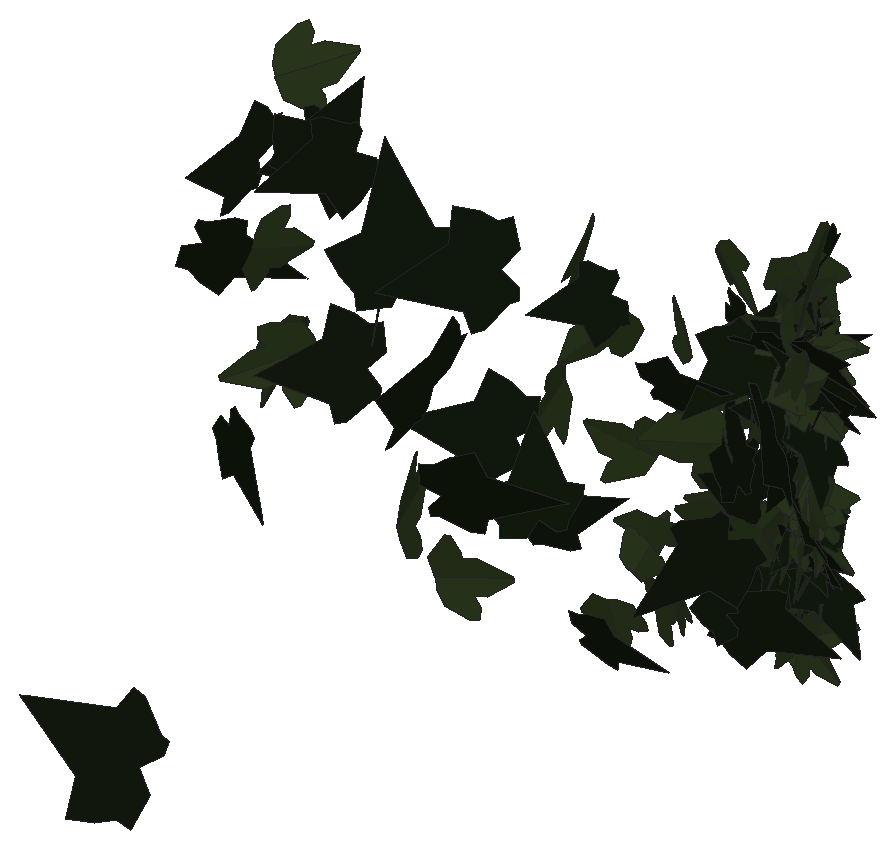
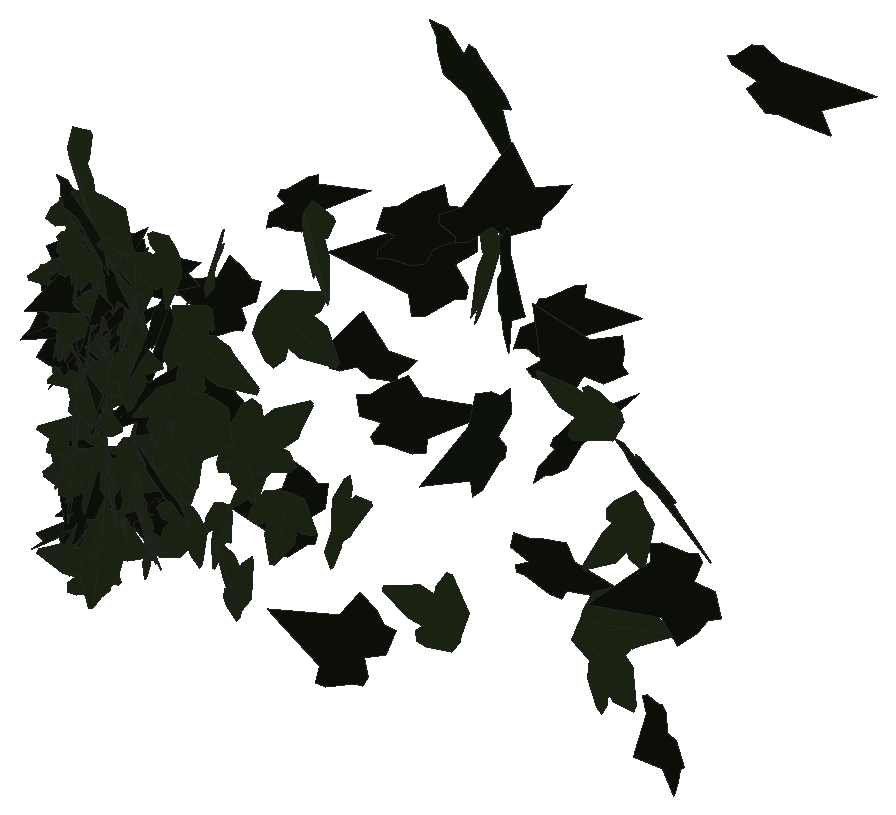
# SketchUp Ruby script. Lengths in inches.
U = 1.inch
M = Sketchup.active_model
def pt(a) = Geom::Point3d.new(a.map { |v| v * U })
def face(e, loops, mat)
  f = e.add_face(loops[0].map { |a| pt(a) })
  loops[1..].each { |l| e.add_face(l.map { |a| pt(a) }).erase! }
  f.material = f.back_material = mat if mat
  f
end
# faces: each face lists its corners as indices into pts; further lists are holes
def faces(e, pts, list, mat = nil) = list.each { |f| face(e, (f[0].is_a?(Array) ? f : [f]).map { |l| l.map { |i| pts[i] } }, mat) }
# xy, xz, yz: faces in a plane at the given z, y or x. An outline is a flat list of corners, or four numbers for a rectangle; further outlines are holes
def ring(l) = l.size == 4 ? [[l[0], l[1]], [l[2], l[1]], [l[2], l[3]], [l[0], l[3]]] : l.each_slice(2).to_a
def flat(e, list, mat, &to3) = list.each { |f| face(e, (f[0].is_a?(Array) ? f : [f]).map { |l| ring(l).map { |u, v| to3.(u, v) } }, mat) }
def xy(e, z, list, mat = nil) = flat(e, list, mat) { |x, y| [x, y, z] }
def xz(e, y, list, mat = nil) = flat(e, list, mat) { |x, z| [x, y, z] }
def yz(e, x, list, mat = nil) = flat(e, list, mat) { |y, z| [x, y, z] }
def lines(e, pts, list) = list.each { |a, b| e.add_line(pt(pts[a]), pt(pts[b])) }
# prism: a flat outline (further loops are holes) pulled along v
def prism(e, loops, v, mat = nil)
  f = face(e, loops, mat); d = Geom::Vector3d.new(v.map { |x| x * U })
  f.pushpull(f.normal.samedirection?(d) ? d.length : -d.length)
end
def box(e, o, s, mat = nil) = prism(e, [[o, [o[0] + s[0], o[1], o[2]], [o[0] + s[0], o[1] + s[1], o[2]], [o[0], o[1] + s[1], o[2]]]], [0, 0, s[2]], mat)
def at(x, y, z, deg = 0) = Geom::Transformation.translation(pt([x, y, z])) * Geom::Transformation.rotation(ORIGIN, Z_AXIS, deg.degrees)
def axes(o, x, y, z) = Geom::Transformation.new([*x, 0, *y, 0, *z, 0, *pt(o).to_a, 1])
def part(name) = M.definitions.add(name)
# library, detail: a bought-in or finely detailed component or shape, given as its bounding box
def library(name, o, s) = part(name).tap { |d| box(d.entities, o, s) }
def detail(e, o, s) = box(e.add_group.entities, o, s)
def put(e, d, t, mat = nil) = e.add_instance(d, t).tap { |i| i.material = mat if mat }
def group(e, t, mat = nil) = e.add_group.tap { |g| g.transformation = t; g.material = mat if mat }.entities
root = M.entities
M.materials.add("efeu1").color = [18, 25, 13]
M.materials.add("efeu2").color = [43, 57, 29]
c1 = part("ivyleaf_9")
p = [[1.54,2.16,1.25],[1.36,2.04,1.19],[-0.21,0.99,0.68],[-0.71,1.11,0.82],[-0.85,0.86,0.67],[-0.8,0.17,0.21],
  [-0.9,-0.01,0.1],[-0.67,-0.16,-0.02],[-0.08,-0.08,-0.05],[-0.03,-0.6,-0.4],[0.65,-0.88,-0.66],[0.83,-0.6,-0.49],
  [1.29,-0.42,-0.43],[1.8125,-0.07,-0.26],[1.21,0.44,0.15]]
faces(c1.entities,p,[[0,1,2,3,4,5,6,7,8,9,10,11,12,13,14]],"efeu1")
c2 = part("ivyleaf_10")
p = [[0,0.5,-0.03],[-0.0625,2.02,-0.43],[-0.19,2.01,-0.46],[-0.54,1.05,-0.29],[-0.52,0.625,-0.18],[-0.83,0.76,-0.28],
  [-1.16,0.64,-0.33],[-1.15,0.33,-0.24],[-0.77,-0.39,0.02],[-0.3,-0.51,0.16],[0.04,-0.48,0.23],[-0.02,2.01,-0.4375],
  [-0.06,2.01,-0.43],[0.04,-0.49,0.23],[0.67,-0.49,0.14],[1.38,0.36,-0.2],[1.375,0.51,-0.24],[0.81,0.65,-0.19],
  [0.62,0.59,-0.15],[0.6,1.09,-0.28],[0.5,1.23,-0.31]]
faces(c2.entities,p,[[0,1,2,3,4,5,6,7,8,9,10],[11,12,0,13,14,15,16,17,18,19,20]],"efeu2")
put(root,c1,axes([582.17,102.53,177.91],[-0.93537,-0.48465,-0.89648],[-0.80042,-0.4038,1.05345],[-0.63079,1.23107,-0.00739]))
put(root,c1,axes([582.29,115.48,184.26],[-0.73247,1.14725,0.43552],[-0.25175,0.35593,-1.361],[-1.20104,-0.77428,0.01967]))
put(root,c2,axes([580.5,116.68,178.94],[-0.03504,0.01507,1.25714],[-0.80764,0.96354,-0.03406],[-0.96351,-0.80822,-0.01717]))
put(root,c1,axes([580.96,117.87,179.3],[0.6414,0.06722,0.97347],[0.97264,0.04951,-0.64427],[-0.07836,1.16473,-0.02879]))
put(root,c1,axes([576.85,121.08,183.4375],[-0.9038,-0.73638,0.60147],[0.47307,0.37156,1.16577],[-0.82475,1.02008,0.00956]))
put(root,c1,axes([581.51,121.23,177.39],[-0.91994,-0.16178,0.29692],[0.29433,0.04052,0.934],[-0.16644,0.96582,0.01055]))
put(root,c1,axes([578.58,123.02,183.34],[-0.59552,-0.39328,0.97343],[-0.81155,-0.53754,-0.71367],[0.66605,-1.00661,0.00079]))
put(root,c1,axes([574.84,123.16,183.46],[-0.4066,0.16227,-1.11029],[1.00642,-0.46946,-0.43717],[-0.49618,-1.0852,0.0231]))
put(root,c1,axes([582.08,122.8,173.05],[0.59099,-0.20629,0.62747],[0.59502,-0.19926,-0.62594],[0.28676,0.83862,0.00563]))
put(root,c1,axes([581.98,123.71,183.42],[-0.03674,-0.4484,-0.69223],[-0.05769,-0.68983,0.4499],[-0.82275,0.06839,-0.00063]))
put(root,c1,axes([578.5,123.73,177.73],[-0.46486,-0.0952,0.97458],[-0.95808,-0.17874,-0.47445],[0.20237,-1.06487,-0.00749]))
put(root,c1,axes([585.64,124.3,176.6],[-0.0035,0.04747,-1.11243],[-0.00157,-1.11244,-0.04746],[-1.11344,0.00142,0.00356]))
put(root,c2,axes([582.25,123.57,173.63],[-0.82414,-0.10409,-0.03694],[0.03705,0.00142,-0.83069],[0.10405,-0.82497,0.00323]))
put(root,c2,axes([576.16,123.99,172.28],[-0.30247,-0.08255,0.97235],[0.90328,0.36153,0.31168],[-0.36927,0.95197,-0.03405]))
put(root,c1,axes([571.91,124.95,183.84],[-0.02923,-0.38443,-0.92473],[-0.056,-0.92304,0.3855],[-0.99988,0.06294,0.00544]))
put(root,c2,axes([582.64,124.8,175.91],[-0.65772,-0.30074,0.20225],[-0.18186,-0.08863,-0.7232],[0.3135,-0.68238,0.0048]))
put(root,c2,axes([580.02,125.125,183.85],[0.45167,-0.99129,0.04723],[0.02824,-0.03903,-1.0893],[0.99201,0.45246,0.00951]))
put(root,c2,axes([582.47,124.46,174.89],[0.20307,0.44166,-0.59525],[0.20821,0.55835,0.4853],[0.71136,-0.2895,0.02788]))
put(root,c1,axes([582.85,124.88,180.375],[0.3547,-0.07925,0.67611],[0.66329,-0.13123,-0.36336],[0.1531,0.75213,0.00784]))
put(root,c1,axes([585.99,126.1,179.18],[0.06523,-0.507,1.17159],[0.16337,-1.16015,-0.51115],[1.26609,0.17582,0.0056]))
put(root,c2,axes([584.38,125.29,178.92],[-0.32504,0.07068,1.22055],[-1.18819,-0.31576,-0.29813],[0.28799,-1.22298,0.14751]))
put(root,c1,axes([585.21,125.39,173.81],[-0.343,-0.79962,0.40835],[0.17244,0.37033,0.87001],[-0.88114,0.38374,0.01131]))
put(root,c2,axes([580.57,125.81,181.18],[-0.41497,-0.51387,0.77483],[-0.48662,-0.60297,-0.66051],[0.79224,-0.63953,0.00015]))
put(root,c2,axes([583.1,125.24,173.72],[-0.6164,0.35233,0.11163],[-0.09557,0.05773,-0.70999],[-0.35702,-0.62376,-0.00266]))
put(root,c1,axes([571.65,125.78,176.58],[-0.85339,0.08103,0.70567],[-0.70238,0.06808,-0.85723],[-0.10583,-1.10527,-0.00107]))
put(root,c1,axes([570.375,125.24,182.8],[-0.58712,-0.05013,0.79979],[0.79707,0.06588,0.58926],[-0.08277,0.98997,0.00129]))
put(root,c2,axes([583.26,125.53,181.48],[-0.39235,0.6292,-0.08563],[-0.05289,0.06793,0.74145],[0.63279,0.3958,0.00888]))
put(root,c1,axes([585.23,125.36,178.03],[-0.1394,-0.60796,0.74109],[0.15988,0.72365,0.62372],[-0.94512,0.21208,-0.0038]))
put(root,c1,axes([585.57,125.2,173.91],[0.10177,0.10772,-0.99977],[0.48767,0.87351,0.14376],[0.87939,-0.49687,0.03598]))
put(root,c1,axes([566.9,125.91,172.87],[-0.18101,-0.05084,-0.95511],[0.94753,0.12305,-0.18612],[0.13046,-0.96429,0.02661]))
put(root,c2,axes([581.23,126.19,177.14],[-0.43596,-0.29641,-0.80312],[-0.66848,-0.44515,0.52716],[-0.53479,0.79806,-0.00425]))
put(root,c2,axes([568.93,126.3,175.9],[0.28392,0.20306,-1.03576],[-0.84049,-0.60529,-0.34906],[-0.63844,0.88715,-0.00108]))
put(root,c2,axes([584.6,125.74,176.125],[-1.12151,-0.23936,0.38892],[-0.38144,-0.07608,-1.14676],[0.25111,-1.18459,-0.00493]))
put(root,c1,axes([584.91,126.36,181.38],[-0.70613,-0.48878,0.24061],[-0.19812,-0.13654,-0.85879],[0.50749,-0.7334,-0.00047]))
put(root,c1,axes([584.99,126.55,176.8],[0.03301,0.04778,0.85129],[-0.62056,-0.58288,0.05678],[0.58471,-0.62132,0.0122]))
put(root,c2,axes([581.64,126.35,172.23],[-0.47915,0.12037,0.77564],[0.75107,-0.19371,0.49403],[0.22805,0.89089,0.00262]))
put(root,c2,axes([583.87,126.32,176.32],[-0.49622,-0.36773,0.31232],[-0.25775,-0.17668,-0.61753],[0.40784,-0.55907,-0.01027]))
put(root,c2,axes([584.49,126.83,173],[-0.12467,0.23622,-0.59228],[0.0462,-0.59856,-0.24845],[-0.63597,-0.08979,0.09805]))
put(root,c2,axes([568.09,125.8125,179.2],[-0.13983,-0.38674,-0.93422],[0.31512,0.87947,-0.41125],[0.96075,-0.34475,-0.00108]))
put(root,c2,axes([584.65,126.98,179.65],[-0.08804,0.30993,-0.6085],[0.1578,-0.5877,-0.32217],[-0.6644,-0.18065,0.00412]))
put(root,c1,axes([567.35,126.4,181.41],[-0.82327,0.75225,0.36065],[-0.29416,0.21237,-1.11449],[-0.78065,-0.87335,0.03962]))
put(root,c1,axes([572.34,126.67,180.68],[0.98632,-0.53087,0.11326],[0.09969,-0.05374,-1.12011],[0.53359,0.99135,-0.00007]))
put(root,c1,axes([569.29,127.62,181.86],[0.2206,-0.71775,-0.75354],[0.2562,-0.70912,0.75044],[-1.00864,-0.3371,0.02581]))
put(root,c1,axes([565.74,126.29,178.21],[0.16963,0.21121,-0.96973],[0.50806,0.82663,0.26891],[0.85256,-0.53463,0.03269]))
put(root,c2,axes([585.58,127.33,172.43],[-0.20273,0.3687,0.76453],[0.34712,-0.68129,0.4206],[0.77457,0.40181,0.01162]))
put(root,c1,axes([584.92,126.46,181.77],[0.67205,0.44331,-0.09212],[-0.08109,-0.04436,-0.80505],[-0.44546,0.67688,0.00757]))
put(root,c2,axes([584.93,127.31,175.88],[-0.07555,-0.4841,0.51265],[-0.08314,-0.50587,-0.48995],[0.70017,-0.1123,-0.00286]))
put(root,c1,axes([585.2,127.7,178.13],[0.34566,-0.34734,-1.02118],[0.843,-0.58198,0.4833],[-0.67291,-0.90751,0.08091]))
put(root,c2,axes([584.92,127.38,173.9],[-0.11298,-0.21399,-0.59135],[0.18528,-0.58548,0.17647],[-0.60097,-0.14027,0.16557]))
put(root,c2,axes([567.78,127.5,175.56],[0.14329,-0.90028,0.5439],[0.13463,-0.52871,-0.91061],[1.04317,0.1919,0.04281]))
put(root,c1,axes([585.65,127.68,179.2],[-0.21749,-0.09841,0.81849],[-0.56861,-0.59501,-0.22263],[0.59691,-0.60266,0.08615]))
put(root,c1,axes([585.92,127.54,176.01],[0.51861,-0.26683,-0.50331],[0.45478,-0.21599,0.58311],[-0.34308,-0.68966,0.01212]))
put(root,c2,axes([576.98,127.84,176.83],[0.00492,0.27558,-1.00343],[-0.01675,-1.00329,-0.27563],[-1.04045,0.01745,-0.00031]))
put(root,c2,axes([584.75,127.12,181.93],[-0.65202,-0.36991,0.09537],[-0.08279,-0.04733,-0.74964],[0.37293,-0.65725,0.00031]))
put(root,c2,axes([584.76,127.26,180.35],[-0.31984,0.04707,-0.60666],[0.55158,-0.26698,-0.31151],[-0.25695,-0.63171,0.08645]))
put(root,c2,axes([585.33,127.53,179.35],[0.18007,-0.1421,0.66759],[0.51689,-0.42252,-0.22935],[0.44576,0.54734,-0.00373]))
put(root,c2,axes([586.35,127.55,184.8],[0.71848,-0.97219,0.35474],[0.20971,-0.28612,-1.20887],[1.01342,0.74846,-0.00135]))
put(root,c2,axes([585.73,127.67,174.77],[0.23607,-0.28493,0.63083],[0.41476,-0.47539,-0.36993],[0.55418,0.47716,0.00814]))
put(root,c2,axes([586.13,127.22,181.3125],[0.01819,-0.89941,-0.16555],[0.08683,0.16653,-0.89521],[0.91038,0.00208,0.08869]))
put(root,c2,axes([584.9,127.24,174.82],[-0.60543,0.32042,-0.18819],[-0.16626,0.08815,0.68499],[0.33232,0.62784,-0.00014]))
put(root,c2,axes([586.0625,127.58,176.98],[0.3499,-0.27622,-0.70319],[0.53936,-0.4513,0.44566],[-0.52902,-0.64283,-0.01072]))
put(root,c2,axes([585.3,126.8,181.07],[0.35422,-0.11,-1.10319],[1.01416,0.50003,0.27578],[0.44789,-1.04521,0.24803]))
put(root,c1,axes([586.17,127.74,178.76],[0.07757,-0.79632,0.18314],[0.08695,-0.17488,-0.79721],[0.81247,0.09474,0.06784]))
put(root,c1,axes([585.55,127.76,174.05],[-0.6011,-0.61068,-0.00073],[0.00064,0.00039,-0.85688],[0.61068,-0.6011,0.00019]))
put(root,c2,axes([585.8,127.43,172.24],[0.23437,-0.07647,0.87599],[0.87838,-0.02155,-0.23689],[0.04065,0.90654,0.06827]))
put(root,c1,axes([586.11,127.72,181.13],[0.04619,0.09351,0.82911],[-0.75499,-0.34881,0.0814],[0.35519,-0.75358,0.0652]))
put(root,c2,axes([584.63,127.4,179.13],[-0.25537,-0.64602,-0.0655],[0.0241,0.0609,-0.69467],[0.64889,-0.25651,0.00002]))
put(root,c2,axes([585.91,127.7,172.6],[0.34664,-0.40429,-0.49776],[0.32326,-0.37851,0.53255],[-0.55382,-0.47398,-0.0007]))
put(root,c2,axes([582.54,127.44,174.71],[-0.66984,0.15741,-0.47062],[0.44423,-0.16215,-0.68652],[-0.22117,-0.80241,0.0464]))
put(root,c2,axes([585.71,127.77,173.63],[0.30358,-0.45476,0.39202],[0.25235,-0.30196,-0.54571],[0.5448,0.39327,0.03432]))
put(root,c2,axes([585.91,127.91,182.83],[-0.02609,-0.00679,-0.69846],[0.32842,-0.61699,-0.00626],[-0.61647,-0.32841,0.02622]))
put(root,c2,axes([585.95,127.8,178.125],[0.23449,-0.53181,0.33498],[0.13606,-0.3061,-0.58121],[0.61361,0.2711,0.00087]))
put(root,c2,axes([585.61,127.39,182.66],[-0.70114,0.21954,0.05595],[-0.05654,0.00667,-0.73463],[-0.21939,-0.70334,0.0105]))
put(root,c2,axes([585.75,127.33,176.54],[0.58017,0.2718,-0.31643],[0.28581,0.13582,0.64068],[0.30385,-0.64674,0.00156]))
put(root,c1,axes([585.98,127.16,181.47],[0.89815,0.2158,0.07116],[0.06818,0.02084,-0.9237],[-0.21676,0.90072,0.00432]))
put(root,c2,axes([585.78,127.01,182.36],[-0.17055,0.3974,0.65637],[-0.23493,0.61305,-0.43222],[-0.73045,-0.28996,-0.01424]))
put(root,c2,axes([582.16,127.24,178.29],[-0.39569,-0.55883,-0.54734],[0.34627,0.42488,-0.68412],[0.7014,-0.52501,0.02896]))
put(root,c1,axes([585.625,127.31,178.97],[-0.3906,-0.56018,0.69726],[0.43529,0.54561,0.68219],[-0.78134,0.584,0.03148]))
put(root,c2,axes([585.75,127.77,172.74],[0.45616,0.3002,-0.35701],[-0.28998,-0.20861,-0.54594],[-0.36536,0.54039,-0.01243]))
put(root,c2,axes([584.61,127.42,181.03],[-0.53886,0.43171,0.14197],[-0.11061,0.089,-0.69046],[-0.44079,-0.55009,-0.0003]))
put(root,c1,axes([576.45,127.45,172.6875],[0.18869,-0.03637,0.96057],[0.96029,-0.03699,-0.19003],[0.04333,0.97823,0.02852]))
put(root,c1,axes([585.69,127.3,180.57],[0.04364,0.01929,-0.8828],[0.34403,0.81366,0.03479],[0.81324,-0.34525,0.03265]))
put(root,c2,axes([585.48,127.35,175.39],[0.25225,-0.40311,-0.78831],[-0.4325,0.65913,-0.47545],[0.77257,0.50061,-0.00877]))
put(root,c2,axes([586.13,127.97,175.98],[-0.07764,0.66866,-0.42249],[0.06,-0.41832,-0.67308],[-0.78867,-0.09765,-0.00961]))
put(root,c2,axes([583.55,128.25,175.12],[0.80071,-0.7352,0.63241],[0.47093,-0.42215,-1.08702],[0.84776,0.92891,0.00653]))
put(root,c2,axes([585.68,127.38,172.13],[-0.18951,-0.2574,0.82414],[0.54654,0.61742,0.31852],[-0.66839,0.57785,0.02678]))
put(root,c1,axes([586.11,128.13,176.1],[-0.70824,-0.31423,0.03925],[-0.03101,-0.02688,-0.77472],[0.31515,-0.70881,0.01198]))
put(root,c2,axes([582.86,127.9,183.09],[-0.47553,0.34572,-0.6184],[0.51911,-0.33683,-0.58748],[-0.48214,-0.70363,-0.02261]))
put(root,c1,axes([586.02,127.6875,182.62],[-0.65779,0.41981,0.37626],[-0.32798,0.18529,-0.78012],[-0.45852,-0.7348,0.01824]))
put(root,c2,axes([586.1,127.86,175.23],[-0.26764,0.0905,-0.62935],[0.59787,-0.19657,-0.28252],[-0.2164,-0.65504,-0.00217]))
put(root,c2,axes([585.78,127.84,182.69],[-0.51391,-0.26927,0.38648],[0.35748,0.1495,0.57951],[-0.30672,0.6254,0.02787]))
put(root,c1,axes([585.65,127.56,175.3],[0.76823,0.21503,-0.3587],[-0.34997,-0.08017,-0.7976],[-0.22896,0.84405,0.01562]))
put(root,c2,axes([585.86,127.39,175.51],[-0.0553,0.4126,0.55173],[-0.06391,0.54805,-0.41625],[-0.68598,-0.08432,-0.00569]))
put(root,c2,axes([585.59,127.82,178.2],[-0.59874,0.00965,-0.22602],[0.225,-0.04102,-0.59779],[-0.02349,-0.63866,0.03498]))
put(root,c1,axes([585.97,128.15,173.79],[0.24836,-0.84997,0.01492],[0.31932,0.07887,-0.8223],[0.78785,0.23597,0.32858]))
put(root,c2,axes([586.15,127.52,181.73],[-0.19233,-0.10663,-0.74464],[0.62342,0.40753,-0.21938],[0.42097,-0.65223,-0.01533]))
put(root,c2,axes([585.2,128.48,178.47],[0.00086,-0.40032,0.7161],[0.09999,-0.71071,-0.39743],[0.81429,0.0877,0.04804]))
put(root,c2,axes([585.15,127.87,175.78],[-0.86459,-0.66925,-0.01567],[0.0133,0.00843,-1.09335],[0.6693,-0.86469,0.00147]))
put(root,c1,axes([585.21,128.2,182.42],[-0.72097,-0.06172,-0.63413],[0.63049,0.06865,-0.72353],[0.09166,-0.95771,-0.011]))
put(root,c1,axes([585.9375,128.14,179.6],[0.6807,0.02336,-0.41472],[0.41395,0.02788,0.681],[0.03445,-0.7966,0.01167]))
put(root,c2,axes([585.77,128.17,180.61],[-0.38269,-0.60302,0.33848],[-0.18102,-0.28601,-0.7142],[0.66741,-0.42335,0.00037]))
put(root,c2,axes([585.95,127.58,179.9],[0.25951,0.62902,0.48722],[0.15291,0.4635,-0.67984],[-0.78081,0.29983,0.0288]))
put(root,c2,axes([586.05,127.8125,176.54],[0.51015,0.53551,0.33474],[0.22388,0.24901,-0.73956],[-0.5905,0.55705,0.00879]))
put(root,c2,axes([585.73,127.68,179.51],[0.13674,-0.40295,-0.49517],[-0.05681,0.49671,-0.41989],[0.63588,0.13103,0.06897]))
put(root,c2,axes([586.02,127.69,178.55],[0.32459,0.75384,-0.27108],[0.1053,0.2498,0.82075],[0.79414,-0.34124,0.00197]))
put(root,c2,axes([585.5,127.875,183.7],[-0.88834,-0.32743,-0.35664],[0.33599,0.11963,-0.94676],[0.34858,-0.94975,0.00369]))
put(root,c2,axes([585.2,127.97,173.59],[-0.6139,-0.75342,-0.13774],[0.08735,0.10651,-0.97186],[0.76091,-0.62008,0.00043]))
put(root,c1,axes([585.35,128.54,174.43],[0.23707,-0.40742,0.82215],[0.41202,-0.71146,-0.47137],[0.81986,0.47536,-0.00085]))
put(root,c2,axes([585.83,128.13,176.32],[0.25742,-0.88053,0.03344],[0.33144,0.06447,-0.85364],[0.81646,0.25145,0.336]))
put(root,c1,axes([585.77,127.42,181.26],[0.39398,0.3852,0.63308],[0.4003,0.49277,-0.54894],[-0.62365,0.55964,0.0476]))
put(root,c2,axes([586.32,127.92,180.39],[-0.15965,-0.62118,-0.28322],[0.07049,0.27431,-0.64137],[0.67905,-0.17452,-0.00001]))
put(root,c2,axes([585.78,128.02,182.6875],[-0.60245,0.25201,-0.0886],[0.07789,-0.04335,-0.65296],[-0.25553,-0.60738,0.00985]))
put(root,c2,axes([567.47,127.98,183.59],[0.53295,-0.22774,-0.89789],[0.92341,0.0486,0.53577],[-0.07334,-1.04301,0.22102]))
put(root,c1,axes([582.86,127.91,175.62],[-0.46699,0.55109,0.3708],[0.24496,-0.27844,0.72232],[0.6174,0.5273,-0.00611]))
put(root,c2,axes([585.02,128.47,182.67],[0.21307,0.45849,-0.49364],[-0.22557,-0.43932,-0.50539],[-0.63484,0.30998,0.01389]))
put(root,c1,axes([583.02,127.98,181.44],[0.60784,-0.35734,-0.42709],[-0.36532,0.2213,-0.70508],[0.42029,0.70916,0.00482]))
put(root,c2,axes([585.875,128.19,180.52],[0.72415,0.24292,0.13779],[0.13077,0.04341,-0.76381],[-0.24676,0.73586,-0.00043]))
put(root,c2,axes([585.78,127.99,177.85],[-0.03434,-0.57818,-0.31718],[0.04445,0.31486,-0.57876],[0.65797,-0.05144,0.02254]))
put(root,c1,axes([585.85,127.65,178.78],[-0.17448,0.53948,0.61049],[-0.17952,0.58353,-0.56696],[-0.79467,-0.25027,-0.00596]))
put(root,c2,axes([585.25,127.6875,181.02],[0.09156,0.17221,-0.64907],[0.19904,0.61867,0.19222],[0.64135,-0.21659,0.03301]))
put(root,c2,axes([582.76,128.07,179.03],[0.08605,0.83931,0.06935],[0.00477,0.06922,-0.84371],[-0.84216,0.08616,0.0023]))
put(root,c2,axes([585.58,128.53,178.99],[-0.30219,0.21575,-0.60387],[0.32911,-0.52075,-0.35074],[-0.55035,-0.42987,0.12182]))
put(root,c2,axes([585.07,128.1875,174],[0.11205,0.63141,-0.04618],[-0.00751,-0.04557,-0.64127],[-0.63305,0.1123,-0.00057]))
put(root,c1,axes([586.09,127.89,183.97],[-0.42634,0.69016,0.2656],[-0.14158,0.22472,-0.81122],[-0.72582,-0.44923,0.00223]))
put(root,c2,axes([585.86,128.18,176.59],[-0.74278,-0.14663,0.04616],[-0.04512,-0.00982,-0.75711],[0.14696,-0.74415,0.0009]))
